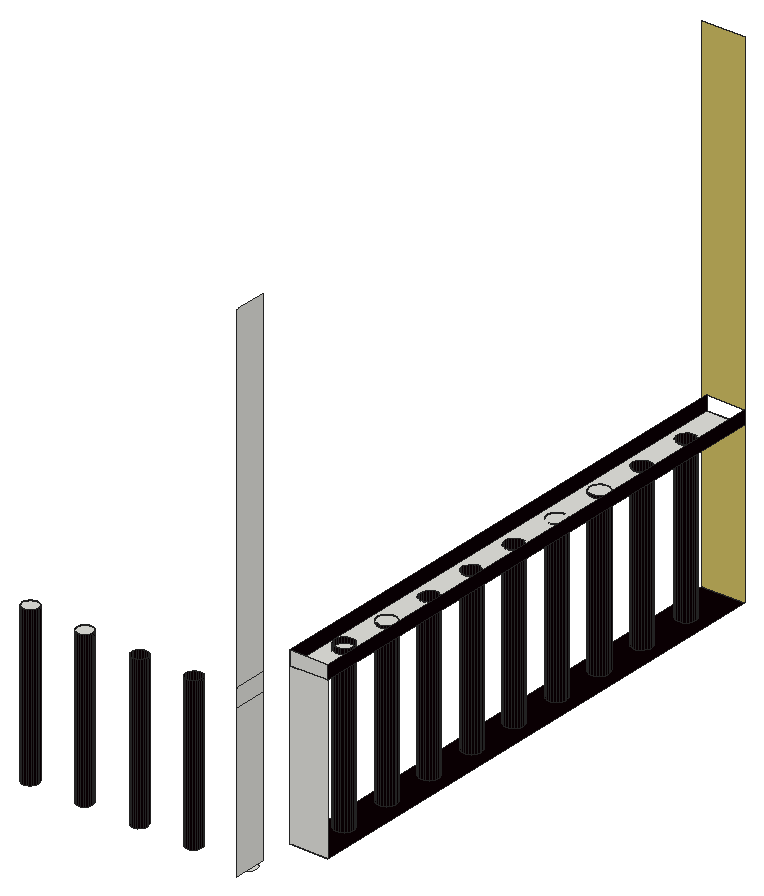
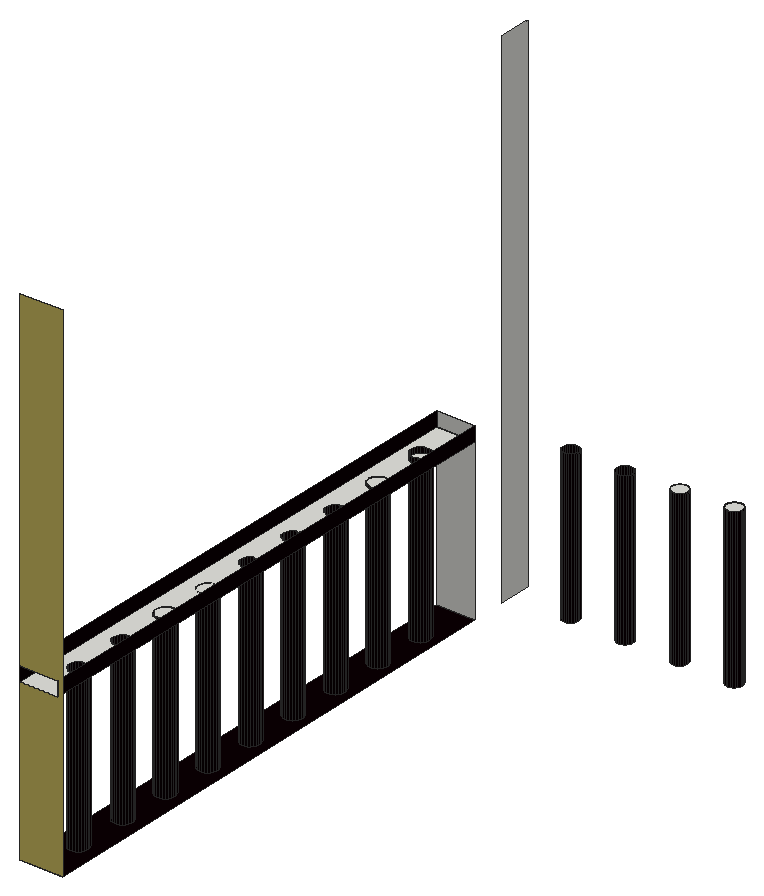
# SketchUp Ruby script. Lengths in inches.
U = 1.inch
M = Sketchup.active_model
def pt(a) = Geom::Point3d.new(a.map { |v| v * U })
def face(e, loops, mat)
  f = e.add_face(loops[0].map { |a| pt(a) })
  loops[1..].each { |l| e.add_face(l.map { |a| pt(a) }).erase! }
  f.material = f.back_material = mat if mat
  f
end
# faces: each face lists its corners as indices into pts; further lists are holes
def faces(e, pts, list, mat = nil) = list.each { |f| face(e, (f[0].is_a?(Array) ? f : [f]).map { |l| l.map { |i| pts[i] } }, mat) }
# xy, xz, yz: faces in a plane at the given z, y or x. An outline is a flat list of corners, or four numbers for a rectangle; further outlines are holes
def ring(l) = l.size == 4 ? [[l[0], l[1]], [l[2], l[1]], [l[2], l[3]], [l[0], l[3]]] : l.each_slice(2).to_a
def flat(e, list, mat, &to3) = list.each { |f| face(e, (f[0].is_a?(Array) ? f : [f]).map { |l| ring(l).map { |u, v| to3.(u, v) } }, mat) }
def xy(e, z, list, mat = nil) = flat(e, list, mat) { |x, y| [x, y, z] }
def xz(e, y, list, mat = nil) = flat(e, list, mat) { |x, z| [x, y, z] }
def yz(e, x, list, mat = nil) = flat(e, list, mat) { |y, z| [x, y, z] }
def lines(e, pts, list) = list.each { |a, b| e.add_line(pt(pts[a]), pt(pts[b])) }
# prism: a flat outline (further loops are holes) pulled along v
def prism(e, loops, v, mat = nil)
  f = face(e, loops, mat); d = Geom::Vector3d.new(v.map { |x| x * U })
  f.pushpull(f.normal.samedirection?(d) ? d.length : -d.length)
end
def box(e, o, s, mat = nil) = prism(e, [[o, [o[0] + s[0], o[1], o[2]], [o[0] + s[0], o[1] + s[1], o[2]], [o[0], o[1] + s[1], o[2]]]], [0, 0, s[2]], mat)
def at(x, y, z, deg = 0) = Geom::Transformation.translation(pt([x, y, z])) * Geom::Transformation.rotation(ORIGIN, Z_AXIS, deg.degrees)
def axes(o, x, y, z) = Geom::Transformation.new([*x, 0, *y, 0, *z, 0, *pt(o).to_a, 1])
def part(name) = M.definitions.add(name)
# library, detail: a bought-in or finely detailed component or shape, given as its bounding box
def library(name, o, s) = part(name).tap { |d| box(d.entities, o, s) }
def detail(e, o, s) = box(e.add_group.entities, o, s)
def put(e, d, t, mat = nil) = e.add_instance(d, t).tap { |i| i.material = mat if mat }
def group(e, t, mat = nil) = e.add_group.tap { |g| g.transformation = t; g.material = mat if mat }.entities
root = M.entities
M.materials.add("[Color D05]").color = [208, 191, 99]
M.materials.add("[Metal Seamed]").color = [11, 0, 4]
xy(root,156,[[532.47,72.62,532.03,72.67,531.62,72.83,531.26,73.09,530.99,73.43,530.8125,73.83,530.75,74.27,530.79,74.71,530.95,75.12,531.21,75.47,531.56,75.75,531.96,75.93,532.4,75.99,532.83,75.94,533.25,75.78,533.6,75.52,533.875,75.18,534.05,74.78,534.12,74.34,534.07,73.9,533.91,73.49,533.65,73.14,533.31,72.86,532.9,72.68],[544.09,72.62,543.66,72.67,543.25,72.83,542.89,73.09,542.61,73.43,542.4375,73.83,542.37,74.27,542.42,74.71,542.58,75.12,542.84,75.47,543.18,75.75,543.59,75.93,544.02,75.99,544.46,75.94,544.87,75.78,545.23,75.52,545.5,75.18,545.68,74.78,545.74,74.34,545.7,73.9,545.54,73.49,545.28,73.14,544.93,72.86,544.53,72.68],[556.3,72.75,556.56,72.86,556.9,73.14,557.16,73.49,557.32,73.9,557.37,74.34,557.3,74.78,557.125,75.18,556.85,75.52,556.5,75.78,556.3,75.86],[559.49,92.73,558.98,92.84,558.52,93.09,558.14,93.44,557.86,93.88,557.7,94.38,557.68,94.9,557.8,95.41,558.04,95.875,558.4,96.26,558.84,96.53,559.34,96.6875,559.86,96.71,560.37,96.59,560.83,96.35,561.22,95.99,561.49,95.55,561.65,95.05,561.67,94.53,561.55,94.02,561.31,93.56,560.95,93.18,560.51,92.9,560.01,92.74],[559.49,104.04,558.98,104.15,558.52,104.4,558.14,104.75,557.86,105.2,557.7,105.69,557.68,106.22,557.8,106.73,558.04,107.1875,558.4,107.57,558.84,107.85,559.34,108,559.86,108.02,560.37,107.9,560.83,107.66,561.22,107.3,561.49,106.86,561.65,106.36,561.67,105.84,561.55,105.33,561.31,104.87,560.95,104.49,560.51,104.21,560.01,104.06],
  [559.49,115.35,558.98,115.47,558.52,115.71,558.14,116.07,557.86,116.51,557.7,117.01,557.68,117.53,557.8,118.04,558.04,118.5,558.4,118.88,558.84,119.16,559.34,119.3125,559.86,119.33,560.37,119.22,560.83,118.97,561.22,118.62,561.49,118.17,561.65,117.68,561.67,117.15,561.55,116.65,561.31,116.18,560.95,115.8,560.51,115.52,560.01,115.37],[559.49,126.66,558.98,126.78,558.52,127.02,558.14,127.38,557.86,127.82,557.7,128.32,557.68,128.84,557.8,129.35,558.04,129.8125,558.4,130.19,558.84,130.47,559.34,130.625,559.86,130.65,560.37,130.53,560.83,130.28,561.22,129.93,561.49,129.49,561.65,128.99,561.67,128.47,561.55,127.96,561.31,127.5,560.95,127.11,560.51,126.84,560.01,126.68],[559.49,137.98,558.98,138.09,558.52,138.34,558.14,138.69,557.86,139.13,557.7,139.63,557.68,140.15,557.8,140.66,558.04,141.125,558.4,141.51,558.84,141.78,559.34,141.9375,559.86,141.96,560.37,141.84,560.83,141.6,561.22,141.24,561.49,140.8,561.65,140.3,561.67,139.78,561.55,139.27,561.31,138.81,560.95,138.43,560.51,138.15,560.01,137.99],[559.49,149.29,558.98,149.4,558.52,149.65,558.14,150,557.86,150.45,557.7,150.94,557.68,151.47,557.8,151.98,558.04,152.4375,558.4,152.82,558.84,153.1,559.34,153.25,559.86,153.27,560.37,153.15,560.83,152.91,561.22,152.55,561.49,152.11,561.65,151.61,561.67,151.09,561.55,150.58,561.31,150.12,560.95,149.74,560.51,149.46,560.01,149.31],[559.49,160.6,558.98,160.72,558.52,160.96,558.14,161.32,557.86,161.76,557.7,162.26,557.68,162.78,557.8,163.29,558.04,163.75,558.4,164.13,558.84,164.41,559.34,164.5625,559.86,164.58,560.37,164.47,560.83,164.22,561.22,163.87,561.49,163.42,561.65,162.93,561.67,162.4,561.55,161.9,561.31,161.43,560.95,161.05,560.51,160.77,560.01,160.62],
  [559.49,171.91,558.98,172.03,558.52,172.27,558.14,172.63,557.86,173.07,557.7,173.57,557.68,174.09,557.8,174.6,558.04,175.0625,558.4,175.44,558.84,175.72,559.34,175.875,559.86,175.9,560.37,175.78,560.83,175.53,561.22,175.18,561.49,174.74,561.65,174.24,561.67,173.72,561.55,173.21,561.31,172.75,560.95,172.36,560.51,172.09,560.01,171.93],[559.49,183.73,558.98,183.84,558.52,184.09,558.14,184.44,557.86,184.88,557.7,185.38,557.68,185.9,557.8,186.41,558.04,186.875,558.4,187.26,558.84,187.53,559.34,187.6875,559.86,187.71,560.37,187.59,560.83,187.35,561.22,186.99,561.49,186.55,561.65,186.05,561.67,185.53,561.55,185.02,561.31,184.56,560.95,184.18,560.51,183.9,560.01,183.74]])
xy(root,156,[[[556.24,84.63,564.3125,84.63,564.3125,195.41,555.3125,195.41],[559.49,92.73,558.98,92.84,558.52,93.09,558.14,93.44,557.86,93.88,557.7,94.38,557.68,94.9,557.8,95.41,558.04,95.875,558.4,96.26,558.84,96.53,559.34,96.6875,559.86,96.71,560.37,96.59,560.83,96.35,561.22,95.99,561.49,95.55,561.65,95.05,561.67,94.53,561.55,94.02,561.31,93.56,560.95,93.18,560.51,92.9,560.01,92.74],[559.49,104.04,558.98,104.15,558.52,104.4,558.14,104.75,557.86,105.2,557.7,105.69,557.68,106.22,557.8,106.73,558.04,107.1875,558.4,107.57,558.84,107.85,559.34,108,559.86,108.02,560.37,107.9,560.83,107.66,561.22,107.3,561.49,106.86,561.65,106.36,561.67,105.84,561.55,105.33,561.31,104.87,560.95,104.49,560.51,104.21,560.01,104.06],[559.49,115.35,558.98,115.47,558.52,115.71,558.14,116.07,557.86,116.51,557.7,117.01,557.68,117.53,557.8,118.04,558.04,118.5,558.4,118.88,558.84,119.16,559.34,119.3125,559.86,119.33,560.37,119.22,560.83,118.97,561.22,118.62,561.49,118.17,561.65,117.68,561.67,117.15,561.55,116.65,561.31,116.18,560.95,115.8,560.51,115.52,560.01,115.37],[559.49,126.66,558.98,126.78,558.52,127.02,558.14,127.38,557.86,127.82,557.7,128.32,557.68,128.84,557.8,129.35,558.04,129.8125,558.4,130.19,558.84,130.47,559.34,130.625,559.86,130.65,560.37,130.53,560.83,130.28,561.22,129.93,561.49,129.49,561.65,128.99,561.67,128.47,561.55,127.96,561.31,127.5,560.95,127.11,560.51,126.84,560.01,126.68],[559.49,137.98,558.98,138.09,558.52,138.34,558.14,138.69,557.86,139.13,557.7,139.63,557.68,140.15,557.8,140.66,558.04,141.125,558.4,141.51,558.84,141.78,559.34,141.9375,559.86,141.96,560.37,141.84,560.83,141.6,561.22,141.24,561.49,140.8,561.65,140.3,561.67,139.78,561.55,139.27,561.31,138.81,560.95,138.43,560.51,138.15,560.01,137.99],[559.49,149.29,558.98,149.4,558.52,149.65,558.14,150,557.86,150.45,557.7,150.94,557.68,151.47,557.8,151.98,558.04,152.4375,558.4,152.82,558.84,153.1,559.34,153.25,559.86,153.27,560.37,153.15,560.83,152.91,561.22,152.55,561.49,152.11,561.65,151.61,561.67,151.09,561.55,150.58,561.31,150.12,560.95,149.74,560.51,149.46,560.01,149.31],[559.49,160.6,558.98,160.72,558.52,160.96,558.14,161.32,557.86,161.76,557.7,162.26,557.68,162.78,557.8,163.29,558.04,163.75,558.4,164.13,558.84,164.41,559.34,164.5625,559.86,164.58,560.37,164.47,560.83,164.22,561.22,163.87,561.49,163.42,561.65,162.93,561.67,162.4,561.55,161.9,561.31,161.43,560.95,161.05,560.51,160.77,560.01,160.62],[559.49,171.91,558.98,172.03,558.52,172.27,558.14,172.63,557.86,173.07,557.7,173.57,557.68,174.09,557.8,174.6,558.04,175.0625,558.4,175.44,558.84,175.72,559.34,175.875,559.86,175.9,560.37,175.78,560.83,175.53,561.22,175.18,561.49,174.74,561.65,174.24,561.67,173.72,561.55,173.21,561.31,172.75,560.95,172.36,560.51,172.09,560.01,171.93],[559.49,183.73,558.98,183.84,558.52,184.09,558.14,184.44,557.86,184.88,557.7,185.38,557.68,185.9,557.8,186.41,558.04,186.875,558.4,187.26,558.84,187.53,559.34,187.6875,559.86,187.71,560.37,187.59,560.83,187.35,561.22,186.99,561.49,186.55,561.65,186.05,561.67,185.53,561.55,185.02,561.31,184.56,560.95,184.18,560.51,183.9,560.01,183.74]]],"[Metal Seamed]")
xy(root,188.8125,[[520.84,72.62,521.28,72.68,521.68,72.86,522.03,73.14,522.29,73.49,522.45,73.9,522.49,74.34,522.43,74.78,522.25,75.18,521.98,75.52,521.62,75.78,521.21,75.94,520.77,75.99,520.34,75.93,519.93,75.75,519.59,75.47,519.33,75.12,519.17,74.71,519.12,74.27,519.1875,73.83,519.36,73.43,519.64,73.09,520,72.83,520.41,72.67]])
xy(root,189.4375,[[509.22,72.62,509.65,72.68,510.06,72.86,510.4,73.14,510.66,73.49,510.82,73.9,510.87,74.34,510.8,74.78,510.625,75.18,510.35,75.52,510,75.78,509.58,75.94,509.15,75.99,508.71,75.93,508.31,75.75,507.96,75.47,507.7,75.12,507.54,74.71,507.5,74.27,507.5625,73.83,507.74,73.43,508.01,73.09,508.37,72.83,508.78,72.67]])
xy(root,189.9375,[[559.49,149.29,560.01,149.31,560.51,149.46,560.95,149.74,561.31,150.12,561.55,150.58,561.67,151.09,561.65,151.61,561.49,152.11,561.22,152.55,560.83,152.91,560.37,153.15,559.86,153.27,559.34,153.25,558.84,153.1,558.4,152.82,558.04,152.4375,557.8,151.98,557.68,151.47,557.7,150.94,557.86,150.45,558.14,150,558.52,149.65,558.98,149.4]])
xy(root,189.95,[[[556.24,84.63,564.3125,195.41],[559.49,115.35,560.01,115.37,560.51,115.52,560.95,115.8,561.31,116.18,561.55,116.65,561.67,117.15,561.65,117.68,561.49,118.17,561.22,118.62,560.83,118.97,560.37,119.22,559.86,119.33,559.34,119.3125,558.84,119.16,558.4,118.88,558.04,118.5,557.8,118.04,557.68,117.53,557.7,117.01,557.86,116.51,558.14,116.07,558.52,115.71,558.98,115.47],[559.49,126.66,560.01,126.68,560.51,126.84,560.95,127.11,561.31,127.5,561.55,127.96,561.67,128.47,561.65,128.99,561.49,129.49,561.22,129.93,560.83,130.28,560.37,130.53,559.86,130.65,559.34,130.625,558.84,130.47,558.4,130.19,558.04,129.8125,557.8,129.35,557.68,128.84,557.7,128.32,557.86,127.82,558.14,127.38,558.52,127.02,558.98,126.78],[559.49,137.98,560.01,137.99,560.51,138.15,560.95,138.43,561.31,138.81,561.55,139.27,561.67,139.78,561.65,140.3,561.49,140.8,561.22,141.24,560.83,141.6,560.37,141.84,559.86,141.96,559.34,141.9375,558.84,141.78,558.4,141.51,558.04,141.125,557.8,140.66,557.68,140.15,557.7,139.63,557.86,139.13,558.14,138.69,558.52,138.34,558.98,138.09],[559.49,171.91,560.01,171.93,560.51,172.09,560.95,172.36,561.31,172.75,561.55,173.21,561.67,173.72,561.65,174.24,561.49,174.74,561.22,175.18,560.83,175.53,560.37,175.78,559.86,175.9,559.34,175.875,558.84,175.72,558.4,175.44,558.04,175.0625,557.8,174.6,557.68,174.09,557.7,173.57,557.86,173.07,558.14,172.63,558.52,172.27,558.98,172.03],[559.49,183.73,560.01,183.74,560.51,183.9,560.95,184.18,561.31,184.56,561.55,185.02,561.67,185.53,561.65,186.05,561.49,186.55,561.22,186.99,560.83,187.35,560.37,187.59,559.86,187.71,559.34,187.6875,558.84,187.53,558.4,187.26,558.04,186.875,557.8,186.41,557.68,185.9,557.7,185.38,557.86,184.88,558.14,184.44,558.52,184.09,558.98,183.84]]])
xy(root,190.375,[[559.49,104.04,560.01,104.06,560.51,104.21,560.95,104.49,561.31,104.87,561.55,105.33,561.67,105.84,561.65,106.36,561.49,106.86,561.22,107.3,560.83,107.66,560.37,107.9,559.86,108.02,559.34,108,558.84,107.85,558.4,107.57,558.04,107.1875,557.8,106.73,557.68,106.22,557.7,105.69,557.86,105.2,558.14,104.75,558.52,104.4,558.98,104.15],[559.49,160.6,560.01,160.62,560.51,160.77,560.95,161.05,561.31,161.43,561.55,161.9,561.67,162.4,561.65,162.93,561.49,163.42,561.22,163.87,560.83,164.22,560.37,164.47,559.86,164.58,559.34,164.5625,558.84,164.41,558.4,164.13,558.04,163.75,557.8,163.29,557.68,162.78,557.7,162.26,557.86,161.76,558.14,161.32,558.52,160.96,558.98,160.72]])
xz(root,70.41,[[556.3,188.2,556.3125,192]])
xz(root,77.3,[[556.3,188.2,556.3125,192]])
xz(root,84.63,[[556.24,156,564.3125,189.95],[556.24,189.95,564.3125,192.96]])
xz(root,195.41,[[555.3125,156,564.3125,156,564.3125,189.95,556.24,189.95,556.24,192.96,564.3125,192.96,564.3125,264,555.3125,264]],"[Color D05]")
yz(root,556.24,[[84.63,189.95,195.41,192.96]],"[Metal Seamed]")
yz(root,556.3,[[70.41,156,70.41,264,70.97,264,70.97,264.0625,77.3,264.0625,77.3,156]])
yz(root,556.3125,[[70.41,188.2,77.3,192]])
yz(root,564.3125,[[84.63,189.95,195.41,192.96]],"[Metal Seamed]")
p = [[508.78,72.67,156],[509.22,72.62,156],[509.22,72.62,189.4375],[508.78,72.67,189.4375],[509.65,72.68,156],[509.65,72.68,189.4375],
  [520.41,72.67,156],[520.84,72.62,156],[520.84,72.62,188.8125],[520.41,72.67,188.8125],[521.28,72.68,156],[521.28,72.68,188.8125],
  [532.03,72.67,156],[532.47,72.62,156],[532.47,72.62,188.2],[532.03,72.67,188.2],[532.9,72.68,156],[532.9,72.68,188.2],
  [543.66,72.67,156],[544.09,72.62,156],[544.09,72.62,188.2],[543.66,72.67,188.2],[544.53,72.68,156],[544.53,72.68,188.2],
  [508.37,72.83,156],[508.37,72.83,189.4375],[510.06,72.86,156],[510.06,72.86,189.4375],[520,72.83,156],[520,72.83,188.8125],
  [521.68,72.86,156],[521.68,72.86,188.8125],[531.62,72.83,156],[531.62,72.83,188.2],[533.31,72.86,156],[533.31,72.86,188.2],
  [543.25,72.83,156],[543.25,72.83,188.2],[544.93,72.86,156],[544.93,72.86,188.2],[508.01,73.09,156],[508.01,73.09,189.4375],
  [519.64,73.09,156],[519.64,73.09,188.8125],[531.26,73.09,156],[531.26,73.09,188.2],[542.89,73.09,156],[542.89,73.09,188.2],
  [510.4,73.14,156],[510.4,73.14,189.4375],[522.03,73.14,156],[522.03,73.14,188.8125],[533.65,73.14,156],[533.65,73.14,188.2],
  [545.28,73.14,156],[545.28,73.14,188.2],[507.74,73.43,156],[507.74,73.43,189.4375],[510.66,73.49,156],[510.66,73.49,189.4375],
  [519.36,73.43,156],[519.36,73.43,188.8125],[522.29,73.49,156],[522.29,73.49,188.8125],[530.99,73.43,156],[530.99,73.43,188.2],
  [533.91,73.49,156],[533.91,73.49,188.2],[542.61,73.43,156],[542.61,73.43,188.2],[545.54,73.49,156],[545.54,73.49,188.2],
  [507.5625,73.83,156],[507.5625,73.83,189.4375],[519.1875,73.83,156],[519.1875,73.83,188.8125],[530.8125,73.83,156],[530.8125,73.83,188.2],
  [542.4375,73.83,156],[542.4375,73.83,188.2],[510.82,73.9,156],[510.82,73.9,189.4375],[522.45,73.9,156],[522.45,73.9,188.8125],
  [534.07,73.9,156],[534.07,73.9,188.2],[545.7,73.9,156],[545.7,73.9,188.2],[507.5,74.27,156],[507.5,74.27,189.4375],
  [519.12,74.27,156],[519.12,74.27,188.8125],[530.75,74.27,156],[530.75,74.27,188.2],[542.37,74.27,156],[542.37,74.27,188.2],
  [510.87,74.34,156],[510.87,74.34,189.4375],[522.49,74.34,156],[522.49,74.34,188.8125],[534.12,74.34,156],[534.12,74.34,188.2],
  [545.74,74.34,156],[545.74,74.34,188.2],[510.8,74.78,156],[510.8,74.78,189.4375],[519.17,74.71,156],[519.17,74.71,188.8125],
  [522.43,74.78,156],[522.43,74.78,188.8125],[530.79,74.71,156],[530.79,74.71,188.2],[534.05,74.78,156],[534.05,74.78,188.2],
  [542.42,74.71,156],[542.42,74.71,188.2],[545.68,74.78,156],[545.68,74.78,188.2],[507.7,75.12,156],[507.54,74.71,156],
  [507.54,74.71,189.4375],[507.7,75.12,189.4375],[519.33,75.12,156],[519.33,75.12,188.8125],[530.95,75.12,156],[530.95,75.12,188.2],
  [542.58,75.12,156],[542.58,75.12,188.2],[510.625,75.18,156],[510.625,75.18,189.4375],[522.25,75.18,156],[522.25,75.18,188.8125],
  [533.875,75.18,156],[533.875,75.18,188.2],[545.5,75.18,156],[545.5,75.18,188.2],[507.96,75.47,156],[507.96,75.47,189.4375],
  [519.59,75.47,156],[519.59,75.47,188.8125],[531.21,75.47,156],[531.21,75.47,188.2],[542.84,75.47,156],[542.84,75.47,188.2],
  [510.35,75.52,156],[510.35,75.52,189.4375],[521.98,75.52,156],[521.98,75.52,188.8125],[533.6,75.52,156],[533.6,75.52,188.2],
  [545.23,75.52,156],[545.23,75.52,188.2],[508.31,75.75,156],[508.31,75.75,189.4375],[510,75.78,156],[510,75.78,189.4375],
  [519.93,75.75,156],[519.93,75.75,188.8125],[521.62,75.78,156],[521.62,75.78,188.8125],[531.56,75.75,156],[531.56,75.75,188.2],
  [533.25,75.78,156],[533.25,75.78,188.2],[543.18,75.75,156],[543.18,75.75,188.2],[544.87,75.78,156],[544.87,75.78,188.2],
  [508.71,75.93,156],[508.71,75.93,189.4375],[520.34,75.93,156],[520.34,75.93,188.8125],[531.96,75.93,156],[531.96,75.93,188.2],
  [543.59,75.93,156],[543.59,75.93,188.2],[509.58,75.94,156],[509.58,75.94,189.4375],[521.21,75.94,156],[521.21,75.94,188.8125],
  [532.83,75.94,156],[532.83,75.94,188.2],[544.46,75.94,156],[544.46,75.94,188.2],[509.15,75.99,156],[509.15,75.99,189.4375],
  [520.77,75.99,156],[520.77,75.99,188.8125],[532.4,75.99,156],[532.4,75.99,188.2],[544.02,75.99,156],[544.02,75.99,188.2],
  [558.98,92.84,156],[559.49,92.73,156],[559.49,92.73,191.0625],[558.98,92.84,191.0625],[560.01,92.74,156],[560.01,92.74,191.0625],
  [560.51,92.9,156],[560.51,92.9,191.0625],[558.52,93.09,156],[558.52,93.09,191.0625],[560.95,93.18,156],[560.95,93.18,191.0625],
  [558.14,93.44,156],[558.14,93.44,191.0625],[561.31,93.56,156],[561.31,93.56,191.0625],[557.86,93.88,156],[557.86,93.88,191.0625],
  [561.55,94.02,156],[561.55,94.02,191.0625],[557.7,94.38,156],[557.7,94.38,191.0625],[561.67,94.53,156],[561.67,94.53,191.0625],
  [557.68,94.9,156],[557.68,94.9,191.0625],[561.65,95.05,156],[561.65,95.05,191.0625],[557.8,95.41,156],[557.8,95.41,191.0625],
  [561.49,95.55,156],[561.49,95.55,191.0625],[558.04,95.875,156],[558.04,95.875,191.0625],[561.22,95.99,156],[561.22,95.99,191.0625],
  [558.4,96.26,156],[558.4,96.26,191.0625],[560.83,96.35,156],[560.83,96.35,191.0625],[558.84,96.53,156],[558.84,96.53,191.0625],
  [560.37,96.59,156],[560.37,96.59,191.0625],[559.34,96.6875,156],[559.34,96.6875,191.0625],[559.86,96.71,156],[559.86,96.71,191.0625],
  [558.98,104.15,156],[559.49,104.04,156],[559.49,104.04,190.375],[558.98,104.15,190.375],[560.01,104.06,156],[560.01,104.06,190.375],
  [560.51,104.21,156],[560.51,104.21,190.375],[558.52,104.4,156],[558.52,104.4,190.375],[560.95,104.49,156],[560.95,104.49,190.375],
  [558.14,104.75,156],[558.14,104.75,190.375],[561.31,104.87,156],[561.31,104.87,190.375],[557.86,105.2,156],[557.86,105.2,190.375],
  [561.55,105.33,156],[561.55,105.33,190.375],[557.7,105.69,156],[557.7,105.69,190.375],[561.67,105.84,156],[561.67,105.84,190.375],
  [557.68,106.22,156],[557.68,106.22,190.375],[561.65,106.36,156],[561.65,106.36,190.375],[557.8,106.73,156],[557.8,106.73,190.375],
  [561.49,106.86,156],[561.49,106.86,190.375],[558.04,107.1875,156],[558.04,107.1875,190.375],[561.22,107.3,156],[561.22,107.3,190.375],
  [558.4,107.57,156],[558.4,107.57,190.375],[560.83,107.66,156],[560.83,107.66,190.375],[558.84,107.85,156],[558.84,107.85,190.375],
  [560.37,107.9,156],[560.37,107.9,190.375],[559.34,108,156],[559.34,108,190.375],[559.86,108.02,156],[559.86,108.02,190.375],
  [558.98,115.47,156],[559.49,115.35,156],[559.49,115.35,189.95],[558.98,115.47,189.95],[560.01,115.37,156],[560.01,115.37,189.95],
  [560.51,115.52,156],[560.51,115.52,189.95],[558.52,115.71,156],[558.52,115.71,189.95],[560.95,115.8,156],[560.95,115.8,189.95],
  [558.14,116.07,156],[558.14,116.07,189.95],[561.31,116.18,156],[561.31,116.18,189.95],[557.86,116.51,156],[557.86,116.51,189.95],
  [561.55,116.65,156],[561.55,116.65,189.95],[557.7,117.01,156],[557.7,117.01,189.95],[561.67,117.15,156],[561.67,117.15,189.95],
  [557.68,117.53,156],[557.68,117.53,189.95],[561.65,117.68,156],[561.65,117.68,189.95],[557.8,118.04,156],[557.8,118.04,189.95],
  [561.49,118.17,156],[561.49,118.17,189.95],[558.04,118.5,156],[558.04,118.5,189.95],[561.22,118.62,156],[561.22,118.62,189.95],
  [558.4,118.88,156],[558.4,118.88,189.95],[560.83,118.97,156],[560.83,118.97,189.95],[558.84,119.16,156],[558.84,119.16,189.95],
  [560.37,119.22,156],[560.37,119.22,189.95],[559.34,119.3125,156],[559.34,119.3125,189.95],[559.86,119.33,156],[559.86,119.33,189.95],
  [558.98,126.78,156],[559.49,126.66,156],[559.49,126.66,189.95],[558.98,126.78,189.95],[560.01,126.68,156],[560.01,126.68,189.95],
  [560.51,126.84,156],[560.51,126.84,189.95],[558.52,127.02,156],[558.52,127.02,189.95],[560.95,127.11,156],[560.95,127.11,189.95],
  [558.14,127.38,156],[558.14,127.38,189.95],[561.31,127.5,156],[561.31,127.5,189.95],[557.86,127.82,156],[557.86,127.82,189.95],
  [561.55,127.96,156],[561.55,127.96,189.95],[557.7,128.32,156],[557.7,128.32,189.95],[561.67,128.47,156],[561.67,128.47,189.95],
  [557.68,128.84,156],[557.68,128.84,189.95],[561.65,128.99,156],[561.65,128.99,189.95],[557.8,129.35,156],[557.8,129.35,189.95],
  [561.49,129.49,156],[561.49,129.49,189.95],[558.04,129.8125,156],[558.04,129.8125,189.95],[561.22,129.93,156],[561.22,129.93,189.95],
  [558.4,130.19,156],[558.4,130.19,189.95],[560.83,130.28,156],[560.83,130.28,189.95],[558.84,130.47,156],[558.84,130.47,189.95],
  [560.37,130.53,156],[560.37,130.53,189.95],[559.34,130.625,156],[559.34,130.625,189.95],[559.86,130.65,156],[559.86,130.65,189.95],
  [558.98,138.09,156],[559.49,137.98,156],[559.49,137.98,189.95],[558.98,138.09,189.95],[560.01,137.99,156],[560.01,137.99,189.95],
  [560.51,138.15,156],[560.51,138.15,189.95],[558.52,138.34,156],[558.52,138.34,189.95],[560.95,138.43,156],[560.95,138.43,189.95],
  [558.14,138.69,156],[558.14,138.69,189.95],[561.31,138.81,156],[561.31,138.81,189.95],[557.86,139.13,156],[557.86,139.13,189.95],
  [561.55,139.27,156],[561.55,139.27,189.95],[557.7,139.63,156],[557.7,139.63,189.95],[561.67,139.78,156],[561.67,139.78,189.95],
  [557.68,140.15,156],[557.68,140.15,189.95],[561.65,140.3,156],[561.65,140.3,189.95],[557.8,140.66,156],[557.8,140.66,189.95],
  [561.49,140.8,156],[561.49,140.8,189.95],[558.04,141.125,156],[558.04,141.125,189.95],[561.22,141.24,156],[561.22,141.24,189.95],
  [558.4,141.51,156],[558.4,141.51,189.95],[560.83,141.6,156],[560.83,141.6,189.95],[558.84,141.78,156],[558.84,141.78,189.95],
  [560.37,141.84,156],[560.37,141.84,189.95],[559.34,141.9375,156],[559.34,141.9375,189.95],[559.86,141.96,156],[559.86,141.96,189.95],
  [558.98,149.4,156],[559.49,149.29,156],[559.49,149.29,189.9375],[558.98,149.4,189.9375],[560.01,149.31,156],[560.01,149.31,189.9375],
  [560.51,149.46,156],[560.51,149.46,189.9375],[558.52,149.65,156],[558.52,149.65,189.9375],[560.95,149.74,156],[560.95,149.74,189.9375],
  [558.14,150,156],[558.14,150,189.9375],[561.31,150.12,156],[561.31,150.12,189.9375],[557.86,150.45,156],[557.86,150.45,189.9375],
  [561.55,150.58,156],[561.55,150.58,189.9375],[557.7,150.94,156],[557.7,150.94,189.9375],[561.67,151.09,156],[561.67,151.09,189.9375],
  [557.68,151.47,156],[557.68,151.47,189.9375],[561.65,151.61,156],[561.65,151.61,189.9375],[557.8,151.98,156],[557.8,151.98,189.9375],
  [561.49,152.11,156],[561.49,152.11,189.9375],[558.04,152.4375,156],[558.04,152.4375,189.9375],[561.22,152.55,156],[561.22,152.55,189.9375],
  [558.4,152.82,156],[558.4,152.82,189.9375],[560.83,152.91,156],[560.83,152.91,189.9375],[558.84,153.1,156],[558.84,153.1,189.9375],
  [560.37,153.15,156],[560.37,153.15,189.9375],[559.34,153.25,156],[559.34,153.25,189.9375],[559.86,153.27,156],[559.86,153.27,189.9375],
  [558.98,160.72,156],[559.49,160.6,156],[559.49,160.6,190.375],[558.98,160.72,190.375],[560.01,160.62,156],[560.01,160.62,190.375],
  [560.51,160.77,156],[560.51,160.77,190.375],[558.52,160.96,156],[558.52,160.96,190.375],[560.95,161.05,156],[560.95,161.05,190.375],
  [558.14,161.32,156],[558.14,161.32,190.375],[561.31,161.43,156],[561.31,161.43,190.375],[557.86,161.76,156],[557.86,161.76,190.375],
  [561.55,161.9,156],[561.55,161.9,190.375],[557.7,162.26,156],[557.7,162.26,190.375],[561.67,162.4,156],[561.67,162.4,190.375],
  [557.68,162.78,156],[557.68,162.78,190.375],[561.65,162.93,156],[561.65,162.93,190.375],[557.8,163.29,156],[557.8,163.29,190.375],
  [561.49,163.42,156],[561.49,163.42,190.375],[558.04,163.75,156],[558.04,163.75,190.375],[561.22,163.87,156],[561.22,163.87,190.375],
  [558.4,164.13,156],[558.4,164.13,190.375],[560.83,164.22,156],[560.83,164.22,190.375],[558.84,164.41,156],[558.84,164.41,190.375],
  [560.37,164.47,156],[560.37,164.47,190.375],[559.34,164.5625,156],[559.34,164.5625,190.375],[559.86,164.58,156],[559.86,164.58,190.375],
  [558.98,172.03,156],[559.49,171.91,156],[559.49,171.91,189.95],[558.98,172.03,189.95],[560.01,171.93,156],[560.01,171.93,189.95],
  [560.51,172.09,156],[560.51,172.09,189.95],[558.52,172.27,156],[558.52,172.27,189.95],[560.95,172.36,156],[560.95,172.36,189.95],
  [558.14,172.63,156],[558.14,172.63,189.95],[561.31,172.75,156],[561.31,172.75,189.95],[557.86,173.07,156],[557.86,173.07,189.95],
  [561.55,173.21,156],[561.55,173.21,189.95],[557.7,173.57,156],[557.7,173.57,189.95],[561.67,173.72,156],[561.67,173.72,189.95],
  [557.68,174.09,156],[557.68,174.09,189.95],[561.65,174.24,156],[561.65,174.24,189.95],[557.8,174.6,156],[557.8,174.6,189.95],
  [561.49,174.74,156],[561.49,174.74,189.95],[558.04,175.0625,156],[558.04,175.0625,189.95],[561.22,175.18,156],[561.22,175.18,189.95],
  [558.4,175.44,156],[558.4,175.44,189.95],[560.83,175.53,156],[560.83,175.53,189.95],[558.84,175.72,156],[558.84,175.72,189.95],
  [560.37,175.78,156],[560.37,175.78,189.95],[559.34,175.875,156],[559.34,175.875,189.95],[559.86,175.9,156],[559.86,175.9,189.95],
  [558.98,183.84,156],[559.49,183.73,156],[559.49,183.73,189.95],[558.98,183.84,189.95],[560.01,183.74,156],[560.01,183.74,189.95],
  [560.51,183.9,156],[560.51,183.9,189.95],[558.52,184.09,156],[558.52,184.09,189.95],[560.95,184.18,156],[560.95,184.18,189.95],
  [558.14,184.44,156],[558.14,184.44,189.95],[561.31,184.56,156],[561.31,184.56,189.95],[557.86,184.88,156],[557.86,184.88,189.95],
  [561.55,185.02,156],[561.55,185.02,189.95],[557.7,185.38,156],[557.7,185.38,189.95],[561.67,185.53,156],[561.67,185.53,189.95],
  [557.68,185.9,156],[557.68,185.9,189.95],[561.65,186.05,156],[561.65,186.05,189.95],[557.8,186.41,156],[557.8,186.41,189.95],
  [561.49,186.55,156],[561.49,186.55,189.95],[558.04,186.875,156],[558.04,186.875,189.95],[561.22,186.99,156],[561.22,186.99,189.95],
  [558.4,187.26,156],[558.4,187.26,189.95],[560.83,187.35,156],[560.83,187.35,189.95],[558.84,187.53,156],[558.84,187.53,189.95],
  [560.37,187.59,156],[560.37,187.59,189.95],[559.34,187.6875,156],[559.34,187.6875,189.95],[559.86,187.71,156],[559.86,187.71,189.95]]
faces(root,p,[[0,1,2,3],[1,4,5,2],[6,7,8,9],[7,10,11,8],[12,13,14,15],[13,16,17,14],[18,19,20,21],[19,22,23,20],
  [24,0,3,25],[4,26,27,5],[28,6,9,29],[10,30,31,11],[32,12,15,33],[16,34,35,17],[36,18,21,37],[22,38,39,23],
  [40,24,25,41],[42,28,29,43],[44,32,33,45],[46,36,37,47],[26,48,49,27],[30,50,51,31],[34,52,53,35],[38,54,55,39],
  [56,40,41,57],[48,58,59,49],[60,42,43,61],[50,62,63,51],[64,44,45,65],[52,66,67,53],[68,46,47,69],[54,70,71,55],
  [72,56,57,73],[74,60,61,75],[76,64,65,77],[78,68,69,79],[58,80,81,59],[62,82,83,63],[66,84,85,67],[70,86,87,71],
  [88,72,73,89],[90,74,75,91],[92,76,77,93],[94,78,79,95],[80,96,97,81],[82,98,99,83],[84,100,101,85],[86,102,103,87],
  [96,104,105,97],[106,90,91,107],[98,108,109,99],[110,92,93,111],[100,112,113,101],[114,94,95,115],[102,116,117,103],[118,119,120,121],
  [122,106,107,123],[124,110,111,125],[126,114,115,127],[104,128,129,105],[108,130,131,109],[112,132,133,113],[116,134,135,117],[136,118,121,137],
  [138,122,123,139],[140,124,125,141],[142,126,127,143],[128,144,145,129],[130,146,147,131],[132,148,149,133],[134,150,151,135],[152,136,137,153],
  [144,154,155,145],[156,138,139,157],[146,158,159,147],[160,140,141,161],[148,162,163,149],[164,142,143,165],[150,166,167,151],[168,152,153,169],
  [170,156,157,171],[172,160,161,173],[174,164,165,175],[154,176,177,155],[158,178,179,159],[162,180,181,163],[166,182,183,167],[184,168,169,185],
  [176,184,185,177],[186,170,171,187],[178,186,187,179],[188,172,173,189],[180,188,189,181],[190,174,175,191],[182,190,191,183],[192,193,194,195],
  [193,196,197,194],[196,198,199,197],[200,192,195,201],[198,202,203,199],[204,200,201,205],[202,206,207,203],[208,204,205,209],[206,210,211,207],
  [212,208,209,213],[210,214,215,211],[216,212,213,217],[214,218,219,215],[220,216,217,221],[218,222,223,219],[224,220,221,225],[222,226,227,223],
  [228,224,225,229],[226,230,231,227],[232,228,229,233],[230,234,235,231],[236,232,233,237],[234,238,239,235],[238,236,237,239],[240,241,242,243],
  [241,244,245,242],[244,246,247,245],[248,240,243,249],[246,250,251,247],[252,248,249,253],[250,254,255,251],[256,252,253,257],[254,258,259,255],
  [260,256,257,261],[258,262,263,259],[264,260,261,265],[262,266,267,263],[268,264,265,269],[266,270,271,267],[272,268,269,273],[270,274,275,271],
  [276,272,273,277],[274,278,279,275],[280,276,277,281],[278,282,283,279],[284,280,281,285],[282,286,287,283],[286,284,285,287],[288,289,290,291],
  [289,292,293,290],[292,294,295,293],[296,288,291,297],[294,298,299,295],[300,296,297,301],[298,302,303,299],[304,300,301,305],[302,306,307,303],
  [308,304,305,309],[306,310,311,307],[312,308,309,313],[310,314,315,311],[316,312,313,317],[314,318,319,315],[320,316,317,321],[318,322,323,319],
  [324,320,321,325],[322,326,327,323],[328,324,325,329],[326,330,331,327],[332,328,329,333],[330,334,335,331],[334,332,333,335],[336,337,338,339],
  [337,340,341,338],[340,342,343,341],[344,336,339,345],[342,346,347,343],[348,344,345,349],[346,350,351,347],[352,348,349,353],[350,354,355,351],
  [356,352,353,357],[354,358,359,355],[360,356,357,361],[358,362,363,359],[364,360,361,365],[362,366,367,363],[368,364,365,369],[366,370,371,367],
  [372,368,369,373],[370,374,375,371],[376,372,373,377],[374,378,379,375],[380,376,377,381],[378,382,383,379],[382,380,381,383],[384,385,386,387],
  [385,388,389,386],[388,390,391,389],[392,384,387,393],[390,394,395,391],[396,392,393,397],[394,398,399,395],[400,396,397,401],[398,402,403,399],
  [404,400,401,405],[402,406,407,403],[408,404,405,409],[406,410,411,407],[412,408,409,413],[410,414,415,411],[416,412,413,417],[414,418,419,415],
  [420,416,417,421],[418,422,423,419],[424,420,421,425],[422,426,427,423],[428,424,425,429],[426,430,431,427],[430,428,429,431],[432,433,434,435],
  [433,436,437,434],[436,438,439,437],[440,432,435,441],[438,442,443,439],[444,440,441,445],[442,446,447,443],[448,444,445,449],[446,450,451,447],
  [452,448,449,453],[450,454,455,451],[456,452,453,457],[454,458,459,455],[460,456,457,461],[458,462,463,459],[464,460,461,465],[462,466,467,463],
  [468,464,465,469],[466,470,471,467],[472,468,469,473],[470,474,475,471],[476,472,473,477],[474,478,479,475],[478,476,477,479],[480,481,482,483],
  [481,484,485,482],[484,486,487,485],[488,480,483,489],[486,490,491,487],[492,488,489,493],[490,494,495,491],[496,492,493,497],[494,498,499,495],
  [500,496,497,501],[498,502,503,499],[504,500,501,505],[502,506,507,503],[508,504,505,509],[506,510,511,507],[512,508,509,513],[510,514,515,511],
  [516,512,513,517],[514,518,519,515],[520,516,517,521],[518,522,523,519],[524,520,521,525],[522,526,527,523],[526,524,525,527],[528,529,530,531],
  [529,532,533,530],[532,534,535,533],[536,528,531,537],[534,538,539,535],[540,536,537,541],[538,542,543,539],[544,540,541,545],[542,546,547,543],
  [548,544,545,549],[546,550,551,547],[552,548,549,553],[550,554,555,551],[556,552,553,557],[554,558,559,555],[560,556,557,561],[558,562,563,559],
  [564,560,561,565],[562,566,567,563],[568,564,565,569],[566,570,571,567],[572,568,569,573],[570,574,575,571],[574,572,573,575],[576,577,578,579],
  [577,580,581,578],[580,582,583,581],[584,576,579,585],[582,586,587,583],[588,584,585,589],[586,590,591,587],[592,588,589,593],[590,594,595,591],
  [596,592,593,597],[594,598,599,595],[600,596,597,601],[598,602,603,599],[604,600,601,605],[602,606,607,603],[608,604,605,609],[606,610,611,607],
  [612,608,609,613],[610,614,615,611],[616,612,613,617],[614,618,619,615],[620,616,617,621],[618,622,623,619],[622,620,621,623]],"[Metal Seamed]")
